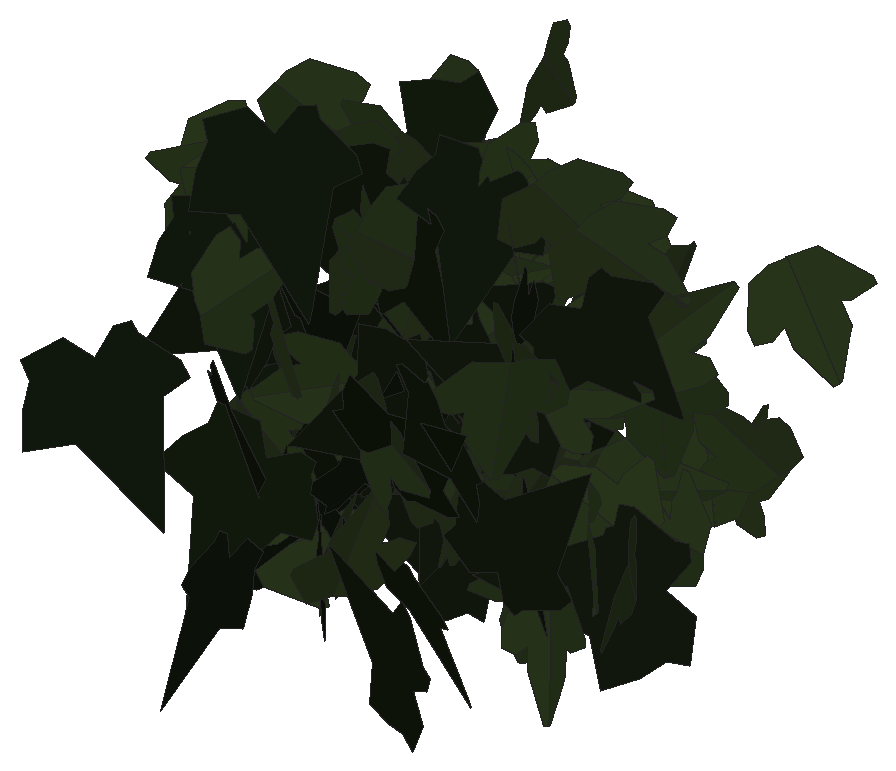
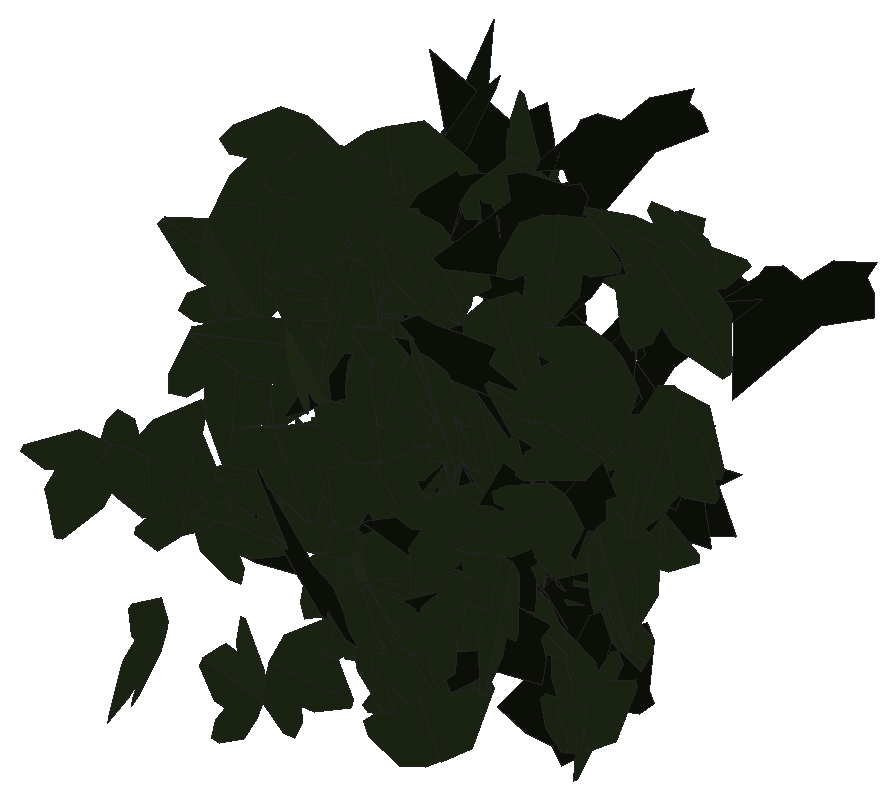
# SketchUp Ruby script. Lengths in inches.
U = 1.inch
M = Sketchup.active_model
def pt(a) = Geom::Point3d.new(a.map { |v| v * U })
def face(e, loops, mat)
  f = e.add_face(loops[0].map { |a| pt(a) })
  loops[1..].each { |l| e.add_face(l.map { |a| pt(a) }).erase! }
  f.material = f.back_material = mat if mat
  f
end
# faces: each face lists its corners as indices into pts; further lists are holes
def faces(e, pts, list, mat = nil) = list.each { |f| face(e, (f[0].is_a?(Array) ? f : [f]).map { |l| l.map { |i| pts[i] } }, mat) }
# xy, xz, yz: faces in a plane at the given z, y or x. An outline is a flat list of corners, or four numbers for a rectangle; further outlines are holes
def ring(l) = l.size == 4 ? [[l[0], l[1]], [l[2], l[1]], [l[2], l[3]], [l[0], l[3]]] : l.each_slice(2).to_a
def flat(e, list, mat, &to3) = list.each { |f| face(e, (f[0].is_a?(Array) ? f : [f]).map { |l| ring(l).map { |u, v| to3.(u, v) } }, mat) }
def xy(e, z, list, mat = nil) = flat(e, list, mat) { |x, y| [x, y, z] }
def xz(e, y, list, mat = nil) = flat(e, list, mat) { |x, z| [x, y, z] }
def yz(e, x, list, mat = nil) = flat(e, list, mat) { |y, z| [x, y, z] }
def lines(e, pts, list) = list.each { |a, b| e.add_line(pt(pts[a]), pt(pts[b])) }
# prism: a flat outline (further loops are holes) pulled along v
def prism(e, loops, v, mat = nil)
  f = face(e, loops, mat); d = Geom::Vector3d.new(v.map { |x| x * U })
  f.pushpull(f.normal.samedirection?(d) ? d.length : -d.length)
end
def box(e, o, s, mat = nil) = prism(e, [[o, [o[0] + s[0], o[1], o[2]], [o[0] + s[0], o[1] + s[1], o[2]], [o[0], o[1] + s[1], o[2]]]], [0, 0, s[2]], mat)
def at(x, y, z, deg = 0) = Geom::Transformation.translation(pt([x, y, z])) * Geom::Transformation.rotation(ORIGIN, Z_AXIS, deg.degrees)
def axes(o, x, y, z) = Geom::Transformation.new([*x, 0, *y, 0, *z, 0, *pt(o).to_a, 1])
def part(name) = M.definitions.add(name)
# library, detail: a bought-in or finely detailed component or shape, given as its bounding box
def library(name, o, s) = part(name).tap { |d| box(d.entities, o, s) }
def detail(e, o, s) = box(e.add_group.entities, o, s)
def put(e, d, t, mat = nil) = e.add_instance(d, t).tap { |i| i.material = mat if mat }
def group(e, t, mat = nil) = e.add_group.tap { |g| g.transformation = t; g.material = mat if mat }.entities
root = M.entities
M.materials.add("efeu1").color = [18, 25, 13]
M.materials.add("efeu2").color = [43, 57, 29]
c1 = part("ivyleaf_10")
p = [[0,0.5,-0.03],[-0.0625,2.02,-0.43],[-0.19,2.01,-0.46],[-0.54,1.05,-0.29],[-0.52,0.625,-0.18],[-0.83,0.76,-0.28],
  [-1.16,0.64,-0.33],[-1.15,0.33,-0.24],[-0.77,-0.39,0.02],[-0.3,-0.51,0.16],[0.04,-0.48,0.23],[-0.02,2.01,-0.4375],
  [-0.06,2.01,-0.43],[0.04,-0.49,0.23],[0.67,-0.49,0.14],[1.38,0.36,-0.2],[1.375,0.51,-0.24],[0.81,0.65,-0.19],
  [0.62,0.59,-0.15],[0.6,1.09,-0.28],[0.5,1.23,-0.31]]
faces(c1.entities,p,[[0,1,2,3,4,5,6,7,8,9,10],[11,12,0,13,14,15,16,17,18,19,20]],"efeu2")
c2 = part("ivyleaf_9")
p = [[1.54,2.16,1.25],[1.36,2.04,1.19],[-0.21,0.99,0.68],[-0.71,1.11,0.82],[-0.85,0.86,0.67],[-0.8,0.17,0.21],
  [-0.9,-0.01,0.1],[-0.67,-0.16,-0.02],[-0.08,-0.08,-0.05],[-0.03,-0.6,-0.4],[0.65,-0.88,-0.66],[0.83,-0.6,-0.49],
  [1.29,-0.42,-0.43],[1.8125,-0.07,-0.26],[1.21,0.44,0.15]]
faces(c2.entities,p,[[0,1,2,3,4,5,6,7,8,9,10,11,12,13,14]],"efeu1")
put(root,c1,axes([525.14,134.7,161.4],[-0.14047,-0.63503,-0.53464],[0.07914,0.52952,-0.64975],[0.82634,-0.15866,-0.02866]))
put(root,c1,axes([525.6,134.35,163.36],[-0.49648,-0.4735,0.44751],[-0.28001,-0.35295,-0.68409],[0.58827,-0.56761,0.05206]))
put(root,c1,axes([524.87,136.84,163.26],[-0.49392,-0.07334,-0.62422],[0.62424,0.03515,-0.49807],[0.07314,-0.79522,0.03556]))
put(root,c1,axes([525.25,135.01,161.08],[-0.64513,-0.34514,-0.25102],[0.2246,0.11231,-0.73162],[0.3629,-0.68307,0.00655]))
put(root,c1,axes([525.39,135.93,159.74],[0.11838,-0.70682,0.06284],[0.01028,-0.062,-0.71666],[0.70953,0.11883,-0.0001]))
put(root,c1,axes([525.13,137.61,161.18],[-0.19191,-0.2351,-0.60549],[0.56788,0.24573,-0.2754],[0.31528,-0.58571,0.12749]))
put(root,c1,axes([525.75,135.65,157.04],[0.02482,0.30738,-0.70426],[-0.01286,0.70469,0.30711],[0.76831,0.00187,0.02789]))
put(root,c1,axes([525.75,135.02,159.42],[-0.36125,-0.66782,-0.07811],[0.03594,0.06937,-0.75926],[0.67141,-0.36303,-0.00139]))
put(root,c1,axes([525.44,136.5,161.68],[0.47106,0.00926,-0.62372],[0.6054,0.18157,0.45993],[0.15033,-0.76024,0.10225]))
put(root,c1,axes([525.72,136.03,156.91],[-0.61089,-0.11009,0.35684],[0.36473,-0.02903,0.61544],[-0.08016,0.70688,0.08084]))
put(root,c1,axes([526.15,137.38,159.53],[-0.65583,0.39283,0.12554],[-0.1099,0.06083,-0.76447],[-0.39749,-0.66496,0.00423]))
put(root,c1,axes([525.44,134.08,163.6],[0.16041,-0.10336,-0.79289],[0.79653,-0.05019,0.16768],[-0.07005,-0.8074,0.09108]))
put(root,c2,axes([526.27,135.6,159.3],[-0.54063,-0.43395,0.31429],[0.2875,0.14181,0.69037],[-0.45214,0.60906,0.06318]))
put(root,c2,axes([525.79,131.11,161.8],[-0.05474,-0.68227,-0.5508],[0.094,0.54413,-0.68334],[0.8718,-0.10151,0.0391]))
put(root,c2,axes([526.07,134.12,161.92],[0.18215,-0.39016,-0.70402],[0.27412,-0.64861,0.43037],[-0.75679,-0.32884,-0.01356]))
put(root,c2,axes([525.92,133.99,162.75],[-0.07969,-0.80622,-0.15795],[0.012,0.15753,-0.81014],[0.82146,-0.08051,-0.00348]))
put(root,c1,axes([526.74,136.35,158.84],[0.13147,-0.05893,-0.79799],[-0.65107,0.46223,-0.14141],[0.46515,0.66364,0.02762]))
put(root,c1,axes([526.22,138.37,159.53],[0.05439,0.0674,-0.67068],[0.14255,0.6565,0.07754],[0.65882,-0.14761,0.0386]))
put(root,c1,axes([525.95,134.54,159.52],[-0.42072,0.13176,-0.54735],[0.51579,-0.18367,-0.44067],[-0.22565,-0.66548,0.01325]))
put(root,c1,axes([526.71,136.67,163.28],[-0.5915,-0.05811,0.38811],[-0.38278,-0.06929,-0.59376],[0.08649,-0.70406,0.0264]))
put(root,c1,axes([526.28,135.15,158.77],[0.04791,-0.78449,-0.11342],[0.03279,-0.11157,0.78553],[-0.79197,-0.05207,0.02567]))
put(root,c2,axes([526.08,135.1875,156.76],[0.56143,0.61805,0.13787],[-0.10558,-0.09031,0.8348],[0.62438,-0.57101,0.0172]))
put(root,c2,axes([526.04,133.88,159.48],[0.10572,-0.22181,0.78729],[0.30316,-0.72667,-0.24544],[0.75968,0.32086,-0.01161]))
put(root,c2,axes([526.39,135.52,159.18],[0.00635,-0.07896,-0.77377],[0.49916,-0.59301,0.06461],[-0.59649,-0.49709,0.04583]))
put(root,c1,axes([526.86,134.04,160.84],[-0.49577,0.53722,-0.37664],[-0.2521,0.27986,0.73101],[0.60573,0.55617,-0.00403]))
put(root,c2,axes([526.48,136.14,158.6875],[-0.32877,-0.69901,-0.15551],[0.07296,0.13753,-0.77243],[0.71237,-0.33669,0.00734]))
put(root,c2,axes([526.18,134.85,160.42],[-0.06244,-0.06848,0.88515],[0.83655,0.29258,0.08165],[-0.29727,0.83773,0.04384]))
put(root,c1,axes([526.6,138.38,163.27],[0.66011,-0.36228,-0.04148],[-0.03654,0.01964,-0.75298],[0.36281,0.66112,-0.00036]))
put(root,c2,axes([526.68,133.71,159.39],[-0.51717,-0.6488,0.02979],[-0.01706,-0.0245,-0.8297],[0.64926,-0.51745,0.00193]))
put(root,c2,axes([526.93,134.6875,157.8],[0.18778,-0.03822,-0.76001],[-0.71489,0.25941,-0.18968],[0.26078,0.73864,0.02729]))
put(root,c1,axes([526.11,134.73,157.4],[0.35095,-0.02681,-0.67078],[0.66908,0.07563,0.34704],[0.05469,-0.75325,0.05872]))
put(root,c1,axes([526.89,135.24,163.92],[-0.45403,-0.52403,-0.1013],[0.06637,0.07653,-0.69336],[0.52959,-0.45886,0.00005]))
put(root,c2,axes([526.6,137.24,158.86],[-0.21869,-0.36976,-0.64994],[0.32905,0.56049,-0.42959],[0.67147,-0.39509,-0.00116]))
put(root,c1,axes([526.46,137.3,159.08],[-0.06429,-0.11668,0.69634],[0.57992,0.39011,0.11892],[-0.40273,0.58037,0.06007]))
put(root,c2,axes([526.29,135.04,158.13],[0.40443,0.01153,-0.68215],[0.6754,0.1053,0.4022],[0.09641,-0.786,0.04388]))
put(root,c2,axes([527.43,137.55,163.1],[-0.77629,-0.06747,0.23343],[-0.23085,-0.03911,-0.77901],[0.07584,-0.80968,0.01818]))
put(root,c1,axes([526.69,137.5,160.51],[0.37283,0.50135,0.35477],[0.21545,0.28188,-0.62477],[-0.57515,0.43059,-0.00406]))
put(root,c2,axes([526.38,136.57,159.5],[0.2909,0.02408,0.75124],[0.74556,0.0929,-0.29167],[-0.09531,0.80022,0.01125]))
put(root,c1,axes([526.79,132.59,162.55],[0.11398,0.09265,-0.75161],[0.32048,0.68276,0.13276],[0.68615,-0.33429,0.06285]))
put(root,c1,axes([527.46,134.47,160.61],[0.34099,-0.00928,-0.69136],[-0.68558,0.09545,-0.33942],[0.08968,0.76495,0.03397]))
put(root,c2,axes([526.51,134.83,161.1875],[-0.05373,-0.21449,0.73979],[0.52832,-0.54991,-0.12106],[0.56051,0.49777,0.18503]))
put(root,c1,axes([526.74,138.4375,158.51],[-0.46159,-0.16084,0.47091],[0.46378,0.09378,0.48663],[-0.18038,0.65271,0.04612]))
put(root,c1,axes([526.97,137.91,157.1],[-0.44948,-0.52311,0.19366],[0.12559,0.14742,0.68969],[-0.54348,0.4667,-0.00079]))
put(root,c1,axes([526.93,136.65,158.28],[0.02233,-0.08227,-0.73938],[0.10863,-0.73143,0.08467],[-0.73597,-0.11046,-0.00994]))
put(root,c1,axes([527.06,134.8125,160.22],[0.41267,-0.64616,0.10611],[-0.05771,0.08905,0.7667],[-0.65227,-0.41668,-0.00071]))
put(root,c1,axes([527.2,134.9,158.17],[0.3561,-0.68384,0.05504],[0.03233,-0.04521,-0.77096],[0.68529,0.35748,0.00777]))
put(root,c2,axes([527.77,135.43,159.29],[-0.27475,0.39585,0.58721],[-0.38569,0.44461,-0.48017],[-0.59393,-0.47184,0.04018]))
put(root,c1,axes([527.54,136.125,161.32],[-0.60148,-0.31617,0.2329],[-0.20496,-0.11063,-0.67951],[0.33496,-0.63544,0.00242]))
put(root,c2,axes([527.29,132.15,158.66],[-0.139,0.19758,-0.73243],[0.46558,-0.56567,-0.24095],[-0.59893,-0.48558,-0.01732]))
put(root,c2,axes([527.17,133.39,164.89],[-0.08358,-0.80538,-0.37116],[0.03635,0.36938,-0.8097],[0.88604,-0.09113,-0.00179]))
put(root,c1,axes([527,135.83,159.64],[-0.11215,-0.08152,0.65502],[0.50405,0.4184,0.13837],[-0.42617,0.5163,-0.00871]))
put(root,c1,axes([527.2,137.125,157.77],[-0.48383,-0.02471,-0.61449],[0.614,0.02478,-0.48445],[0.03476,-0.78171,0.00407]))
put(root,c2,axes([527.2,134.44,163.6875],[0.15001,0.02576,-0.76784],[0.36754,0.6846,0.09478],[0.67465,-0.37869,0.1191]))
put(root,c1,axes([527.52,136.5625,158.5],[0.53326,-0.32469,0.41377],[0.37191,-0.18386,-0.6236],[0.3719,0.64944,0.03032]))
put(root,c2,axes([527.29,135.42,161.49],[0.54458,-0.47213,0.31437],[0.23682,-0.20674,-0.72074],[0.51541,0.59384,-0.00099]))
put(root,c2,axes([528.12,136.5625,157.21],[0.00438,-0.74572,-0.21046],[0.02725,-0.21019,0.74531],[-0.77437,-0.01161,0.02503]))
put(root,c1,axes([527.61,137.69,162.73],[0.6425,0.0441,0.3558],[0.35532,0.01901,-0.64399],[-0.04779,0.73419,-0.0047]))
put(root,c1,axes([528.03,138.41,164.22],[0.07977,-0.54033,-0.43857],[0.03822,0.44417,-0.54029],[0.69487,0.0376,0.08006]))
put(root,c1,axes([528.4,135.8125,160.49],[-0.46719,0.29563,0.57155],[-0.50058,0.27684,-0.55238],[-0.40433,-0.68433,0.02345]))
put(root,c1,axes([528.35,137.51,158.48],[-0.6951,-0.22351,0.24764],[-0.23344,-0.08297,-0.73012],[0.23831,-0.73322,0.00713]))
put(root,c1,axes([528,136.43,161.29],[0.65108,-0.31542,0.15064],[0.13755,-0.06158,-0.72344],[0.32134,0.66543,0.00446]))
put(root,c1,axes([528.06,133.87,157.98],[-0.22688,-0.75915,0.11242],[0.05992,0.09935,0.79181],[-0.76508,0.2329,0.02868]))
put(root,c1,axes([528.18,134.26,162.85],[-0.32144,0.53957,0.45116],[0.21775,-0.39533,0.62794],[0.66878,0.38805,0.0124]))
put(root,c1,axes([528.625,136.97,161.62],[-0.12701,-0.47422,0.54553],[-0.13417,-0.5288,-0.49091],[0.71027,-0.18469,0.00481]))
put(root,c1,axes([528.49,137.28,161.16],[-0.29307,-0.67097,-0.04109],[-0.01621,-0.03776,0.73218],[-0.67203,0.29352,0.00026]))
put(root,c1,axes([528.42,134.03,163.51],[-0.25589,-0.55271,-0.66852],[0.30565,0.59484,-0.60879],[0.81178,-0.3982,0.01849]))
put(root,c1,axes([528.68,139.11,161.73],[0.62723,0.29443,-0.13824],[-0.12572,-0.05749,-0.6929],[-0.29998,0.63971,0.00135]))
put(root,c2,axes([528.18,134.9,163.18],[-0.09953,-0.1287,-0.80002],[0.78821,0.17158,-0.12567],[0.18795,-0.78772,0.10334]))
put(root,c1,axes([529.1,136.58,160.08],[-0.52586,-0.28656,0.45055],[-0.39645,-0.21406,-0.59887],[0.35768,-0.65856,-0.00139]))
put(root,c1,axes([528.77,138.86,157.91],[-0.02199,-0.40986,0.57044],[0.03419,-0.57067,-0.4087],[0.70158,0.01496,0.0378]))
put(root,c1,axes([529.14,136.21,163.62],[0.53134,-0.02957,-0.57194],[-0.56757,0.07698,-0.53127],[0.07646,0.77686,0.03087]))
put(root,c2,axes([528.3125,134.8125,157.68],[0.45462,-0.57454,0.27098],[0.16937,-0.21153,-0.73265],[0.61224,0.48515,0.00146]))
put(root,c2,axes([528.78,136.03,159.64],[-0.34185,-0.74582,0.11068],[-0.04481,-0.10121,-0.82043],[0.75265,-0.34477,0.00143]))
put(root,c2,axes([528.59,138.3,158.83],[-0.34546,0.50343,0.53288],[0.30027,-0.44023,0.61056],[0.66876,0.45771,0.00114]))
put(root,c1,axes([529.02,139.52,157.77],[0.22879,-0.49458,0.48892],[-0.17636,0.45661,0.54443],[-0.67272,-0.28791,0.02356]))
put(root,c1,axes([528.92,135.35,160.73],[0.65893,0.02388,-0.25657],[0.25636,0.01044,0.65936],[0.02604,-0.70704,0.00107]))
put(root,c1,axes([528.9375,135.12,162.35],[-0.0475,-0.0901,0.69977],[0.29231,0.63582,0.10171],[-0.64215,0.29609,-0.00547]))
put(root,c1,axes([529.07,135.99,163.66],[-0.01727,-0.28581,-0.75932],[0.33803,0.6879,-0.26662],[0.73756,-0.32196,0.10441]))
put(root,c2,axes([529.13,135.72,163.81],[-0.18838,-0.78177,0.09077],[-0.02163,-0.08816,-0.80415],[0.78673,-0.18962,-0.00037]))
put(root,c2,axes([529.05,133.1,160.26],[0.39998,0.59419,0.45948],[-0.25602,-0.38155,0.71627],[0.70615,-0.4749,-0.00057]))
put(root,c1,axes([529.39,135.42,159.47],[0.14078,-0.54058,0.47041],[0.10142,-0.45955,-0.55845],[0.70939,0.17298,-0.01351]))
put(root,c2,axes([529.33,135.24,161.84],[0.04093,-0.11735,-0.80752],[0.09383,0.80385,-0.11206],[0.81059,-0.08713,0.05375]))
put(root,c2,axes([529.86,133.04,157.23],[0.12169,-0.79302,0.30633],[-0.00222,0.30916,0.80122],[-0.85013,-0.11432,0.04176]))
put(root,c1,axes([529.51,135.66,161.92],[0.16202,0.2122,-0.76491],[0.32967,0.69219,0.26186],[0.72211,-0.36362,0.05208]))
put(root,c1,axes([529.69,137.48,162.27],[0.28537,-0.58316,0.33017],[0.14812,-0.2951,-0.64923],[0.65357,0.32151,0.00297]))
put(root,c2,axes([529.89,132.94,161.8],[-0.20112,-0.32158,0.7086],[-0.37875,-0.59888,-0.37929],[0.67976,-0.42884,-0.00168]))
put(root,c1,axes([529.5625,136.23,157.15],[0.18685,-0.71932,-0.25458],[0.14265,-0.22455,0.73917],[-0.74958,-0.22204,0.07721]))
put(root,c1,axes([530.17,135.02,162.86],[0.24327,-0.34808,-0.70701],[-0.27117,0.65777,-0.41714],[0.73993,0.3555,0.07958]))
put(root,c1,axes([529.88,135.82,159.64],[-0.28665,-0.63728,-0.08889],[-0.01162,-0.09217,0.69826],[-0.64334,0.28561,0.027]))
put(root,c1,axes([530.13,135.76,157.81],[-0.4623,-0.54099,0.17519],[-0.10718,-0.13885,-0.71156],[0.55845,-0.47449,0.00847]))
put(root,c1,axes([530.07,136.375,158.72],[-0.20787,-0.64513,-0.35991],[-0.12345,-0.33829,0.67768],[-0.72834,0.24146,-0.01214]))
put(root,c1,axes([529.95,136.34,159.47],[0.03402,-0.40387,-0.6787],[0.04762,-0.67704,0.40527],[-0.78833,-0.05832,-0.00481]))
put(root,c1,axes([529.74,133.61,160.25],[-0.48254,0.06416,-0.54493],[0.53822,-0.08582,-0.4867],[-0.10674,-0.7228,0.00942]))
put(root,c1,axes([530.49,135.2,160.16],[-0.15581,-0.49359,0.55589],[-0.13162,-0.54068,-0.51698],[0.73166,-0.20238,0.02538]))
put(root,c1,axes([530.2,135.84,163.98],[-0.57011,-0.40213,-0.4742],[0.38029,0.28346,-0.69759],[0.49189,-0.68523,-0.01029]))
put(root,c1,axes([530.39,133.8,160.3],[-0.0847,-0.41304,-0.77746],[0.22804,0.7441,-0.42016],[0.85032,-0.24069,0.03523]))
put(root,c1,axes([530.07,135.46,160.69],[0.42414,-0.03663,-0.54328],[0.54451,0.02951,0.42311],[0.00077,-0.6886,0.04703]))
put(root,c2,axes([530.82,134.74,161.3125],[-0.06003,-0.7725,-0.20296],[-0.01653,-0.20228,0.77483],[-0.79854,0.06226,-0.00078]))
put(root,c1,axes([530.74,139.49,158.01],[-0.09838,0.20672,0.71004],[-0.32395,0.63187,-0.22884],[-0.66479,-0.3385,0.00644]))
put(root,c2,axes([530.34,135.07,162.63],[-0.11024,0.03209,-0.77064],[0.67992,-0.36351,-0.11239],[-0.36417,-0.6884,0.02343]))
put(root,c2,axes([530.26,134.82,159.76],[-0.0705,-0.00203,-0.79199],[0.79054,-0.04845,-0.07024],[-0.04808,-0.79365,0.00631]))
put(root,c1,axes([530.33,135.93,159.07],[0.54393,-0.12841,0.58758],[0.57553,-0.11891,-0.55876],[0.17464,0.79181,0.01138]))
put(root,c1,axes([530.66,135.18,160.29],[0.14439,-0.28787,0.75953],[0.28583,-0.70408,-0.3212],[0.7603,0.31937,-0.0235]))
put(root,c1,axes([530.33,131.625,162.11],[-0.00926,-0.057,0.84856],[0.83187,-0.17714,-0.00282],[0.17692,0.82992,0.05767]))
put(root,c1,axes([530.4375,136.1,161.31],[0.102,0.05757,-0.87793],[0.778,0.40681,0.11707],[0.41085,-0.78464,-0.00372]))
put(root,c1,axes([531.26,135.99,158.93],[0.3079,0.46074,0.52889],[-0.2903,-0.4421,0.55414],[0.63853,-0.42316,-0.0031]))
put(root,c2,axes([530.625,131.64,161.74],[-0.08371,-0.1865,0.8269],[0.64451,-0.55372,-0.05964],[0.55059,0.61982,0.19553]))
put(root,c1,axes([531.74,136.93,158.46],[0.08295,0.10844,0.7082],[-0.70617,-0.10803,0.09925],[0.12099,-0.70481,0.09375]))
put(root,c1,axes([530.91,136.36,159.31],[-0.15096,-0.11057,-0.78905],[0.5621,0.55439,-0.18523],[0.56469,-0.58141,-0.02656]))
put(root,c1,axes([530.8,134.22,162.05],[-0.34029,0.06535,0.7255],[0.70258,-0.18204,0.34593],[0.19238,0.78039,0.01994]))
put(root,c2,axes([531.99,135.97,158.21],[-0.31632,-0.41834,-0.72366],[-0.38337,-0.61496,0.52307],[-0.74278,0.49555,0.0382]))
put(root,c1,axes([531.56,133.11,162.67],[-0.50746,-0.6926,0.08549],[-0.04316,-0.07435,-0.85856],[0.69652,-0.50921,0.00909]))
put(root,c1,axes([530.875,134.75,161.57],[-0.14133,-0.09611,0.7972],[0.68017,0.41588,0.17072],[-0.42676,0.69465,0.00808]))
put(root,c1,axes([531.17,140.1,161.04],[0.5149,0.46528,0.31846],[0.23748,0.21218,-0.69398],[-0.51138,0.56702,-0.00163]))
put(root,c1,axes([531.6,136.53,161.1],[-0.59048,-0.56812,-0.02613],[0.01903,0.01791,-0.81941],[0.5684,-0.59079,0.00029]))
put(root,c1,axes([531.6,137.59,158.84],[0.1916,0.71191,-0.07057],[0.01765,0.06833,0.73724],[0.71518,-0.19241,0.00071]))
put(root,c1,axes([531.6,136.84,162.89],[0.16518,-0.67439,0.30094],[0.0655,-0.29378,-0.6943],[0.73558,0.1776,-0.00575]))
put(root,c1,axes([531.36,134.22,158.41],[0.71149,-0.17134,0.27035],[0.26449,-0.05634,-0.7318],[0.18024,0.75903,0.0067]))
put(root,c1,axes([531.39,135.39,163.88],[-0.50967,-0.32549,-0.57879],[0.48244,0.31984,-0.60469],[0.45628,-0.70176,-0.00715]))
put(root,c2,axes([531.36,131.93,162.39],[0.54176,-0.44276,-0.44674],[0.35252,-0.27456,0.69962],[-0.52091,-0.64629,0.00884]))
put(root,c2,axes([531.4,133.18,159.61],[-0.29923,0.15401,0.72475],[0.62054,-0.37501,0.33589],[0.40487,0.6886,0.02083]))
put(root,c1,axes([532.22,138,159.48],[-0.50035,-0.20557,-0.47401],[-0.43231,-0.19476,0.54081],[-0.28293,0.66114,0.01192]))
put(root,c2,axes([531.64,134.77,163.08],[0.01595,-0.34438,-0.6838],[0.02924,0.68372,-0.34366],[0.76507,-0.01896,0.02739]))
put(root,c1,axes([531.67,135.94,161.86],[-0.29985,-0.50047,0.6204],[0.30317,0.54142,0.58329],[-0.73719,0.42623,-0.01246]))
put(root,c1,axes([532.16,135.02,159.01],[0.20328,-0.57872,-0.52433],[-0.10549,0.51648,-0.61096],[0.77376,0.22245,0.05445]))
